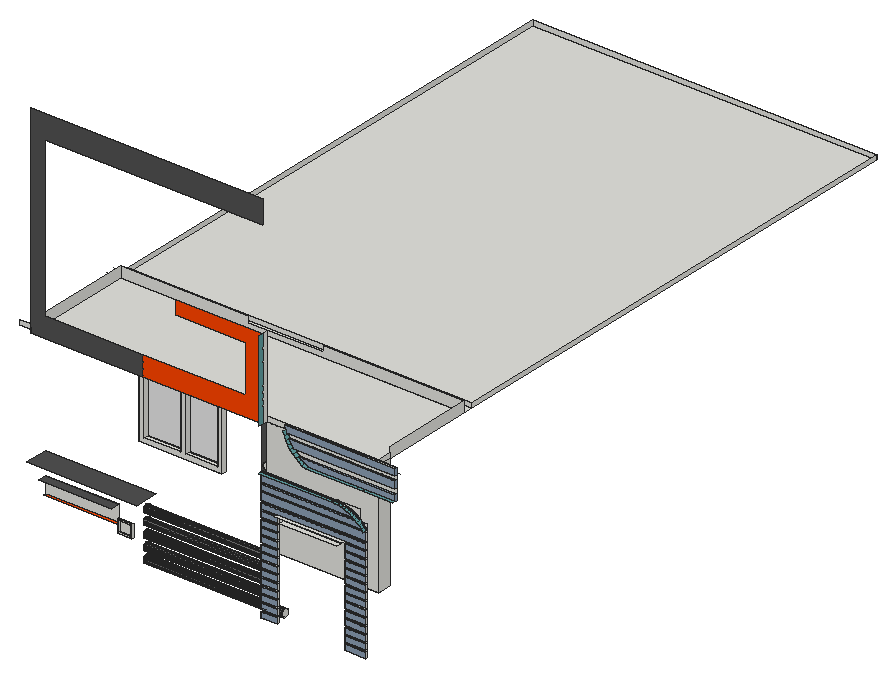
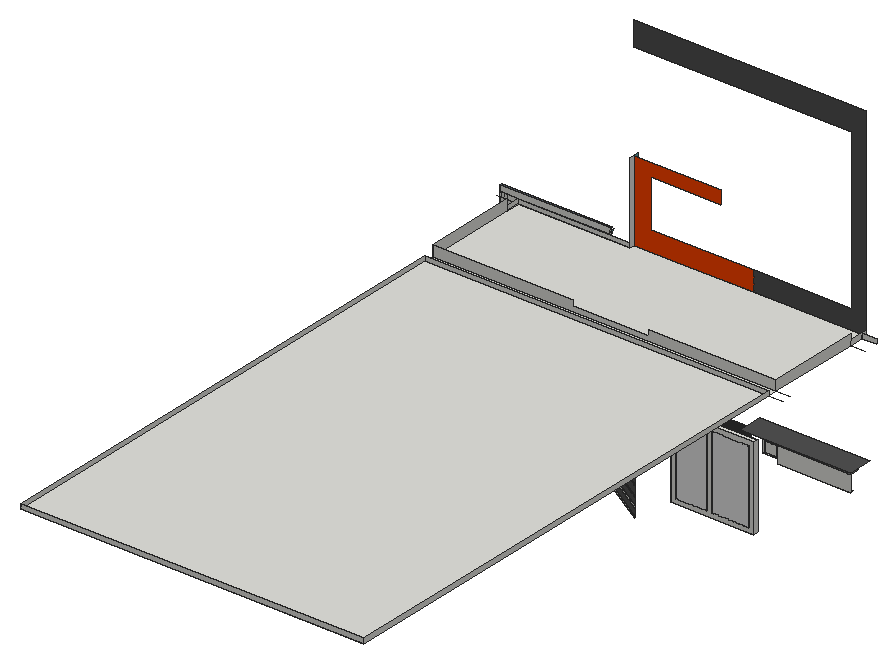
# SketchUp Ruby script. Lengths in inches.
U = 1.inch
M = Sketchup.active_model
def pt(a) = Geom::Point3d.new(a.map { |v| v * U })
def face(e, loops, mat)
  f = e.add_face(loops[0].map { |a| pt(a) })
  loops[1..].each { |l| e.add_face(l.map { |a| pt(a) }).erase! }
  f.material = f.back_material = mat if mat
  f
end
# faces: each face lists its corners as indices into pts; further lists are holes
def faces(e, pts, list, mat = nil) = list.each { |f| face(e, (f[0].is_a?(Array) ? f : [f]).map { |l| l.map { |i| pts[i] } }, mat) }
# xy, xz, yz: faces in a plane at the given z, y or x. An outline is a flat list of corners, or four numbers for a rectangle; further outlines are holes
def ring(l) = l.size == 4 ? [[l[0], l[1]], [l[2], l[1]], [l[2], l[3]], [l[0], l[3]]] : l.each_slice(2).to_a
def flat(e, list, mat, &to3) = list.each { |f| face(e, (f[0].is_a?(Array) ? f : [f]).map { |l| ring(l).map { |u, v| to3.(u, v) } }, mat) }
def xy(e, z, list, mat = nil) = flat(e, list, mat) { |x, y| [x, y, z] }
def xz(e, y, list, mat = nil) = flat(e, list, mat) { |x, z| [x, y, z] }
def yz(e, x, list, mat = nil) = flat(e, list, mat) { |y, z| [x, y, z] }
def lines(e, pts, list) = list.each { |a, b| e.add_line(pt(pts[a]), pt(pts[b])) }
# prism: a flat outline (further loops are holes) pulled along v
def prism(e, loops, v, mat = nil)
  f = face(e, loops, mat); d = Geom::Vector3d.new(v.map { |x| x * U })
  f.pushpull(f.normal.samedirection?(d) ? d.length : -d.length)
end
def box(e, o, s, mat = nil) = prism(e, [[o, [o[0] + s[0], o[1], o[2]], [o[0] + s[0], o[1] + s[1], o[2]], [o[0], o[1] + s[1], o[2]]]], [0, 0, s[2]], mat)
def at(x, y, z, deg = 0) = Geom::Transformation.translation(pt([x, y, z])) * Geom::Transformation.rotation(ORIGIN, Z_AXIS, deg.degrees)
def axes(o, x, y, z) = Geom::Transformation.new([*x, 0, *y, 0, *z, 0, *pt(o).to_a, 1])
def part(name) = M.definitions.add(name)
# library, detail: a bought-in or finely detailed component or shape, given as its bounding box
def library(name, o, s) = part(name).tap { |d| box(d.entities, o, s) }
def detail(e, o, s) = box(e.add_group.entities, o, s)
def put(e, d, t, mat = nil) = e.add_instance(d, t).tap { |i| i.material = mat if mat }
def group(e, t, mat = nil) = e.add_group.tap { |g| g.transformation = t; g.material = mat if mat }.entities
root = M.entities
M.materials.add("[0024_OrangeRed]").color = [255, 69, 0]
M.materials.add("[0081_CadetBlue]").color = [95, 158, 160]
M.materials.add("[0110_LightSlateGray]").color = [139, 158, 178]
M.materials.add("[0134_DimGray]").color = [105, 105, 105]
M.materials.add("[0135_DarkGray]").color = [81, 81, 81]
M.materials.add("[Mirror 02]").color = [229, 229, 229]
xy(root,130.6875,[[213.13,8,226.59,9]])
xy(root,130.6875,[[160.53,8,170.69,9]],"[0110_LightSlateGray]")
xy(root,134.07,[[160.53,8,170.69,9],[213.13,8,226.59,9]],"[0110_LightSlateGray]")
xy(root,135.43,[[213.13,8,226.59,9]])
xy(root,135.43,[[160.53,8,170.69,9]],"[0110_LightSlateGray]")
xy(root,138.8125,[[160.53,8,170.69,9],[213.13,8,226.59,9]],"[0110_LightSlateGray]")
xy(root,140.17,[[213.13,8,226.59,9]])
xy(root,140.17,[[160.53,8,170.69,9]],"[0110_LightSlateGray]")
xy(root,143.55,[[160.53,8,170.69,9],[213.13,8,226.59,9]],"[0110_LightSlateGray]")
xy(root,144.92,[[213.13,8,226.59,9]])
xy(root,144.92,[[160.53,8,170.69,9]],"[0110_LightSlateGray]")
xy(root,148.3,[[160.53,8,170.69,9],[213.13,8,226.59,9]],"[0110_LightSlateGray]")
xy(root,148.91,[[72,5,81.25,6]])
xy(root,149.66,[[213.13,8,226.59,9]])
xy(root,149.66,[[160.53,8,170.69,9]],"[0110_LightSlateGray]")
xy(root,149.71,[[72.8,5,80.45,6]])
xy(root,150.3,[[21.23,10.125,67.5,12]],"[0024_OrangeRed]")
xy(root,153.04,[[160.53,8,170.69,9],[213.13,8,226.59,9]],"[0110_LightSlateGray]")
xy(root,153.81,[[28.3,76.875,80.67,79.875]])
xy(root,154.4,[[213.13,8,226.59,9]])
xy(root,154.4,[[160.53,8,170.69,9]],"[0110_LightSlateGray]")
xy(root,156.24,[[72.8,5,80.45,6]])
xy(root,156.81,[[31.3,76.875,54.48,79.875],[57.67,76.875,77.67,79.875]])
xy(root,157.04,[[72,5,81.25,6]])
xy(root,157.78,[[160.53,8,170.69,9],[213.13,8,226.59,9]],"[0110_LightSlateGray]")
xy(root,159.14,[[213.13,8,226.59,9]])
xy(root,159.14,[[160.53,8,170.69,9]],"[0110_LightSlateGray]")
xy(root,160.4375,[[21.23,6,67.5,12]],"[0135_DarkGray]")
xy(root,162.52,[[160.53,8,170.69,9],[213.13,8,226.59,9]],"[0110_LightSlateGray]")
xy(root,163.88,[[213.13,8,226.59,9]])
xy(root,163.88,[[160.53,8,170.69,9]],"[0110_LightSlateGray]")
xy(root,167.26,[[160.53,8,170.69,9],[213.13,8,226.59,9]],"[0110_LightSlateGray]")
xy(root,168,[[160.53,12,231.375,21]])
xy(root,168,[[14,6,83.4375,21]],"[0135_DarkGray]")
xy(root,168.625,[[213.13,8,226.59,9]])
xy(root,168.625,[[160.53,8,170.69,9]],"[0110_LightSlateGray]")
xy(root,172.01,[[160.53,8,170.69,9],[213.13,8,226.59,9]],"[0110_LightSlateGray]")
xy(root,173.37,[[213.13,8,226.59,9]])
xy(root,173.37,[[160.53,8,170.69,9]],"[0110_LightSlateGray]")
xy(root,176.75,[[160.53,8,170.69,9],[213.13,8,226.59,9]],"[0110_LightSlateGray]")
xy(root,178.11,[[213.13,8,226.59,9]])
xy(root,178.11,[[160.53,8,170.69,9]],"[0110_LightSlateGray]")
xy(root,181.49,[[160.53,8,170.69,9],[213.13,8,226.59,9]],"[0110_LightSlateGray]")
xy(root,182.85,[[213.13,8,226.59,9]])
xy(root,182.85,[[160.53,8,170.69,9]],"[0110_LightSlateGray]")
xy(root,186.23,[[160.53,8,170.69,9],[213.13,8,226.59,9]],"[0110_LightSlateGray]")
xy(root,187.59,[[213.13,8,226.59,9]])
xy(root,187.59,[[160.53,8,170.69,9]],"[0110_LightSlateGray]")
xy(root,189.37,[[173.69,6,210.13,9]])
xy(root,190.98,[[160.53,8,170.69,9],[213.13,8,226.59,9]],"[0110_LightSlateGray]")
xy(root,192.34,[[170.69,6,213.13,9],[213.13,8,226.59,9]])
xy(root,192.34,[[160.53,8,170.69,9]],"[0110_LightSlateGray]")
xy(root,192.37,[[170.69,8,213.13,9]])
xy(root,195.72,[[160.53,8,226.59,9]],"[0110_LightSlateGray]")
xy(root,197.1,[[160.53,8,226.59,9]],"[0110_LightSlateGray]")
xy(root,201,[[105.55,73.875,147.55,76.875]],"[0135_DarkGray]")
xy(root,201.62,[[160.53,8,226.59,9]],"[0110_LightSlateGray]")
xy(root,202.88,[[160.53,8,226.59,9]],"[0110_LightSlateGray]")
xy(root,203.18,[[31.3,76.875,54.48,79.875],[57.67,76.875,77.67,79.875]])
xy(root,204,[[102.55,73.875,150.55,79.875]],"[0135_DarkGray]")
xy(root,206.18,[[28.3,76.875,80.67,79.875]])
xy(root,206.57,[[160.53,8,223.35,9]],"[0110_LightSlateGray]")
xy(root,207.78,[[160.53,8,221.97,9]],"[0110_LightSlateGray]")
xy(root,213.14,[[160.53,8,206.79,9]])
xy(root,213.14,[[160.53,6,206.79,8]],"[0081_CadetBlue]")
xy(root,226.28,[[190.26,8,226.59,9],[226.59,8,245.1875,9]])
xy(root,226.28,[[190.26,6,226.59,8],[226.59,6,240.375,8],[240.375,6,245.1875,8]],"[0081_CadetBlue]")
xy(root,230.16,[[183.95,8,245.1875,9]],"[0110_LightSlateGray]")
xy(root,233.27,[[180.84,8,245.1875,9]],"[0110_LightSlateGray]")
xy(root,237.82,[[177.75,8,245.1875,9]],"[0110_LightSlateGray]")
xy(root,240,[[14,9,14,79.875,231.375,79.875,231.375,12,160.53,12,160.53,9],[14,79.875,231.375,85.875],[14,85.875,231.375,405.4375]])
xy(root,240.67,[[176.48,8,245.1875,9]],"[0110_LightSlateGray]")
xz(root,5,[[[72,148.91,81.25,157.04],[72.8,149.71,80.45,156.24]]])
xz(root,6,[[72.8,149.71,80.45,156.24]])
xz(root,8,[[160.53,130.6875,170.69,134.07],[213.13,130.6875,226.59,134.07],[160.53,135.43,170.69,138.8125],[213.13,135.43,226.59,138.8125],[160.53,140.17,170.69,143.55],
  [213.13,140.17,226.59,143.55],[160.53,144.92,170.69,148.3],[213.13,144.92,226.59,148.3],[160.53,149.66,170.69,153.04],[213.13,149.66,226.59,153.04],
  [160.53,154.4,170.69,157.78],[213.13,154.4,226.59,157.78],[160.53,159.14,170.69,162.52],[213.13,159.14,226.59,162.52],[160.53,163.88,170.69,167.26],
  [213.13,163.88,226.59,167.26],[160.53,168.625,170.69,172.01],[213.13,168.625,226.59,172.01],[160.53,173.37,170.69,176.75],[213.13,173.37,226.59,176.75],
  [160.53,178.11,170.69,181.49],[213.13,178.11,226.59,181.49],[160.53,182.85,170.69,186.23],[213.13,182.85,226.59,186.23],[160.53,187.59,170.69,190.98],
  [213.13,187.59,226.59,190.98],[160.53,192.34,170.69,192.34,170.69,192.37,213.13,192.37,213.13,192.34,226.59,192.34,226.59,195.72,160.53,195.72],[160.53,197.1,226.59,201.62],[160.53,202.88,226.59,202.88,225.42,204.41,224.12,205.84,223.35,206.57,160.53,206.57],[160.53,207.78,221.97,207.78,221.22,208.38,219.62,209.47,217.94,210.42,216.19,211.24,214.39,211.92,212.53,212.45,210.64,212.84,208.72,213.07,206.79,213.14,160.53,213.14],
  [190.26,226.28,245.1875,226.28,245.1875,230.16,183.95,230.16,185.92,228.66,188.03,227.37],[180.84,233.27,245.1875,233.27,245.1875,237.82,177.75,237.82,179.01,235.68,180.47,233.68],[176.48,240.67,245.1875,240.67,245.1875,244.8,175.28,244.8,175.87,242.4]],"[0110_LightSlateGray]")
xz(root,9,[[160.53,130.6875,170.69,134.07],[213.13,130.6875,226.59,134.07],[160.53,134.07,170.69,135.43],[213.13,134.07,226.59,135.43],[160.53,135.43,170.69,138.8125],
  [213.13,135.43,226.59,138.8125],[160.53,138.8125,170.69,140.17],[213.13,138.8125,226.59,140.17],[160.53,140.17,170.69,143.55],[213.13,140.17,226.59,143.55],
  [160.53,143.55,170.69,144.92],[213.13,143.55,226.59,144.92],[160.53,144.92,170.69,148.3],[213.13,144.92,226.59,148.3],[160.53,148.3,170.69,149.66],
  [213.13,148.3,226.59,149.66],[160.53,149.66,170.69,153.04],[213.13,149.66,226.59,153.04],[160.53,153.04,170.69,154.4],[213.13,153.04,226.59,154.4],
  [160.53,154.4,170.69,157.78],[213.13,154.4,226.59,157.78],[160.53,157.78,170.69,159.14],[213.13,157.78,226.59,159.14],[160.53,159.14,170.69,162.52],
  [213.13,159.14,226.59,162.52],[160.53,162.52,170.69,163.88],[213.13,162.52,226.59,163.88],[160.53,163.88,170.69,167.26],[213.13,163.88,226.59,167.26],
  [160.53,167.26,170.69,168.625],[213.13,167.26,226.59,168.625],[160.53,168.625,170.69,172.01],[213.13,168.625,226.59,172.01],[160.53,172.01,170.69,173.37],
  [213.13,172.01,226.59,173.37],[160.53,173.37,170.69,176.75],[213.13,173.37,226.59,176.75],[160.53,176.75,170.69,178.11],[213.13,176.75,226.59,178.11],
  [160.53,178.11,170.69,181.49],[213.13,178.11,226.59,181.49],[160.53,181.49,170.69,182.85],[213.13,181.49,226.59,182.85],[160.53,182.85,170.69,186.23],
  [213.13,182.85,226.59,186.23],[160.53,186.23,170.69,187.59],[213.13,186.23,226.59,187.59],[160.53,187.59,170.69,190.98],[213.13,187.59,226.59,190.98],
  [160.53,190.98,170.69,192.34],[213.13,190.98,226.59,192.34],[160.53,192.34,160.53,195.72,226.59,195.72,226.59,192.34,213.13,192.34,213.13,192.37,170.69,192.37,170.69,192.34],[170.69,192.34,213.13,192.37],[160.53,195.72,226.59,197.1],
  [160.53,197.1,226.59,201.62],[160.53,201.62,226.59,202.88],[160.53,202.88,160.53,206.57,223.35,206.57,224.12,205.84,225.42,204.41,226.59,202.88],[226.59,202.88,226.59,206.57,223.35,206.57,224.12,205.84,225.42,204.41],[160.53,206.57,223.35,206.57,222.72,207.17,221.97,207.78,160.53,207.78],
  [160.53,207.78,160.53,213.14,206.79,213.14,208.72,213.07,210.64,212.84,212.53,212.45,214.39,211.92,216.19,211.24,217.94,210.42,219.62,209.47,221.22,208.38,221.97,207.78],[221.97,207.78,221.97,213.14,206.79,213.14,208.72,213.07,210.64,212.84,212.53,212.45,214.39,211.92,216.19,211.24,217.94,210.42,219.62,209.47,221.22,208.38],[183.95,226.28,190.26,226.28,188.03,227.37,185.92,228.66,183.95,230.16],[190.26,226.28,188.03,227.37,185.92,228.66,183.95,230.16,245.1875,230.16,245.1875,226.28],[183.95,230.16,245.1875,230.16,245.1875,233.27,180.84,233.27,182.125,231.84],
  [177.75,233.27,180.84,233.27,180.47,233.68,179.01,235.68,177.75,237.82],[180.84,233.27,180.47,233.68,179.01,235.68,177.75,237.82,245.1875,237.82,245.1875,233.27],[177.75,237.82,245.1875,237.82,245.1875,240.67,176.48,240.67,176.7,240.0625],[175.28,240.67,176.48,240.67,175.87,242.4,175.28,244.8],[176.48,240.67,175.87,242.4,175.28,244.8,245.1875,244.8,245.1875,240.67]])
xz(root,9,[[85.04,240,160.53,240,160.53,291,105.73,291,105.73,282.37,150.17,282.37,150.17,252.44,85.04,252.44]],"[0024_OrangeRed]")
xz(root,9,[[14,240,85.04,240,85.04,252.44,22.75,252.44,22.75,352.5,160.53,352.5,160.53,367.625,14,367.625]],"[0135_DarkGray]")
xz(root,12,[[21.23,150.3,67.5,160.4375],[160.53,168,231.375,240],[5,240,14,243],[160.53,240,231.375,243],[231.375,240,238.75,243],
  [238.75,240,240.375,243],[240.375,240,241.9375,243]])
xz(root,73.875,[[111.2,167.51,111.84,167.53,112.45,167.71,112.99,168.05,113.42,168.52,113.72,169.08,113.86,169.7,113.84,170.34,113.65,170.94,113.3125,171.48,112.85,171.92,112.29,172.22,111.67,172.36,111.03,172.34,110.42,172.15,109.88,171.8125,109.45,171.35,109.15,170.78,109.01,170.16,109.03,169.53,109.22,168.92,109.55,168.38,110.02,167.95,110.58,167.65]])
xz(root,76.875,[[105.55,134.71,147.55,171.23,147.55,172.96,105.55,135.64],[105.55,140.71,147.55,177.23,147.55,178.96,105.55,141.64],[105.55,146.71,147.55,183.23,147.55,184.96,105.55,147.64],[105.55,152.71,147.55,189.23,147.55,190.96,105.55,153.64],[[28.3,153.81,80.67,206.18],[31.3,156.81,54.48,203.18],[57.67,156.81,77.67,203.18]]])
xz(root,76.875,[[105.55,135.64,147.55,172.96,147.55,177.23,105.55,140.71],[105.55,141.64,147.55,178.96,147.55,183.23,105.55,146.71],[105.55,147.64,147.55,184.96,147.55,189.23,105.55,152.71],[[105.55,153.64,147.55,190.96,147.55,201,105.55,201],[111.2,167.51,110.58,167.65,110.02,167.95,109.55,168.38,109.22,168.92,109.03,169.53,109.01,170.16,109.15,170.78,109.45,171.35,109.88,171.8125,110.42,172.15,111.03,172.34,111.67,172.36,112.29,172.22,112.85,171.92,113.3125,171.48,113.65,170.94,113.84,170.34,113.86,169.7,113.72,169.08,113.42,168.52,112.99,168.05,112.45,167.71,111.84,167.53]]],"[0135_DarkGray]")
xz(root,79.875,[[[28.3,153.81,80.67,206.18],[31.3,156.81,54.48,203.18],[57.67,156.81,77.67,203.18]],[14,240,231.375,240,231.375,246.6875,142.49,246.6875,142.49,243,94.49,243,94.49,246.6875,14,246.6875]])
xz(root,79.875,[[31.3,156.81,54.48,203.18],[57.67,156.81,77.67,203.18]],"[Mirror 02]")
xz(root,85.875,[[14,240,231.375,243]])
xz(root,405.4375,[[14,240,231.375,243]])
yz(root,14,[[9,240,12,243],[12,240,21,243],[21,240,79.875,246.6875],[85.875,240,405.4375,243]])
yz(root,28.3,[[76.875,153.81,79.875,206.18]])
yz(root,31.3,[[76.875,156.81,79.875,203.18]])
yz(root,54.48,[[76.875,156.81,79.875,203.18]])
yz(root,57.67,[[76.875,156.81,79.875,203.18]])
yz(root,72,[[5,148.91,6,157.04]])
yz(root,72.8,[[5,149.71,6,156.24]])
yz(root,77.67,[[76.875,156.81,79.875,203.18]])
yz(root,80.45,[[5,149.71,6,156.24]])
yz(root,80.67,[[76.875,153.81,79.875,206.18]])
yz(root,81.25,[[5,148.91,6,157.04]])
yz(root,160.53,[[9,240,12,291]])
yz(root,160.53,[[6,240,9,291]],"[0081_CadetBlue]")
yz(root,160.53,[[8,130.6875,9,134.07],[8,135.43,9,138.8125],[8,140.17,9,143.55],[8,144.92,9,148.3],[8,149.66,9,153.04],
  [8,154.4,9,157.78],[8,159.14,9,162.52],[8,163.88,9,167.26],[8,168.625,9,172.01],[8,173.37,9,176.75],
  [8,178.11,9,181.49],[8,182.85,9,186.23],[8,187.59,9,190.98],[8,192.34,9,195.72],[8,197.1,9,201.62],
  [8,202.88,9,206.57],[8,207.78,9,213.14]],"[0110_LightSlateGray]")
yz(root,163.375,[[13.48,160.8125,14.06,160.89,14.6,161.11,15.07,161.47,15.42,161.9375,15.65,162.48,15.73,163.0625,15.65,163.64,15.42,164.1875,15.07,164.65,14.6,165.01,14.06,165.23,13.48,165.3125,12.89,165.23,12.35,165.01,11.88,164.65,11.53,164.1875,11.3,163.64,11.23,163.0625,11.3,162.48,11.53,161.9375,11.88,161.47,12.35,161.11,12.89,160.89]])
yz(root,164.1875,[[13.48,153.6875,14.06,153.76,14.6,153.99,15.07,154.34,15.42,154.8125,15.65,155.35,15.73,155.9375,15.65,156.52,15.42,157.0625,15.07,157.53,14.6,157.88,14.06,158.11,13.48,158.1875,12.89,158.11,12.35,157.88,11.88,157.53,11.53,157.0625,11.3,156.52,11.23,155.9375,11.3,155.35,11.53,154.8125,11.88,154.34,12.35,153.99,12.89,153.76]])
yz(root,164.4375,[[13.48,146.5625,14.06,146.64,14.6,146.86,15.07,147.22,15.42,147.6875,15.65,148.23,15.73,148.8125,15.65,149.39,15.42,149.9375,15.07,150.4,14.6,150.76,14.06,150.98,13.48,151.0625,12.89,150.98,12.35,150.76,11.88,150.4,11.53,149.9375,11.3,149.39,11.23,148.8125,11.3,148.23,11.53,147.6875,11.88,147.22,12.35,146.86,12.89,146.64]])
yz(root,164.6875,[[13.48,139.4375,14.06,139.51,14.6,139.74,15.07,140.09,15.42,140.5625,15.65,141.1,15.73,141.6875,15.65,142.27,15.42,142.8125,15.07,143.28,14.6,143.63,14.06,143.86,13.48,143.9375,12.89,143.86,12.35,143.63,11.88,143.28,11.53,142.8125,11.3,142.27,11.23,141.6875,11.3,141.1,11.53,140.5625,11.88,140.09,12.35,139.74,12.89,139.51]])
yz(root,170.69,[[8,130.6875,9,134.07],[8,135.43,9,138.8125],[8,140.17,9,143.55],[8,144.92,9,148.3],[8,149.66,9,153.04],
  [8,154.4,9,157.78],[8,159.14,9,162.52],[8,163.88,9,167.26],[8,168.625,9,172.01],[8,173.37,9,176.75],
  [8,178.11,9,181.49],[8,182.85,9,186.23],[8,187.59,9,190.98],[8,192.34,9,192.37]])
yz(root,171.375,[[13.48,132.3125,14.06,132.39,14.6,132.61,15.07,132.97,15.42,133.4375,15.65,133.98,15.73,134.5625,15.65,135.14,15.42,135.6875,15.07,136.15,14.6,136.51,14.06,136.73,13.48,136.8125,12.89,136.73,12.35,136.51,11.88,136.15,11.53,135.6875,11.3,135.14,11.23,134.5625,11.3,133.98,11.53,133.4375,11.88,132.97,12.35,132.61,12.89,132.39]])
yz(root,213.13,[[8,130.6875,9,134.07],[8,135.43,9,138.8125],[8,140.17,9,143.55],[8,144.92,9,148.3],[8,149.66,9,153.04],
  [8,154.4,9,157.78],[8,159.14,9,162.52],[8,163.88,9,167.26],[8,168.625,9,172.01],[8,173.37,9,176.75],
  [8,178.11,9,181.49],[8,182.85,9,186.23],[8,187.59,9,190.98],[8,192.34,9,192.37]])
yz(root,226.59,[[8,130.6875,9,134.07],[8,135.43,9,138.8125],[8,140.17,9,143.55],[8,144.92,9,148.3],[8,149.66,9,153.04],
  [8,154.4,9,157.78],[8,159.14,9,162.52],[8,163.88,9,167.26],[8,168.625,9,172.01],[8,173.37,9,176.75],
  [8,178.11,9,181.49],[8,182.85,9,186.23],[8,187.59,9,190.98],[8,192.34,9,195.72],[8,197.1,9,201.62]])
yz(root,231.375,[[12,168,21,240],[12,240,21,243],[21,240,79.875,246.6875],[85.875,240,405.4375,243]])
yz(root,245.1875,[[8,226.28,9,230.16],[8,233.27,9,237.82],[8,240.67,9,244.8]],"[0110_LightSlateGray]")
p = [[83.4375,12.89,132.39],[83.4375,13.48,132.3125],[171.375,13.48,132.3125],[171.375,12.89,132.39],[83.4375,14.06,132.39],[171.375,14.06,132.39],
  [83.4375,12.35,132.61],[171.375,12.35,132.61],[83.4375,14.6,132.61],[171.375,14.6,132.61],[83.4375,11.88,132.97],[171.375,11.88,132.97],
  [83.4375,15.07,132.97],[171.375,15.07,132.97],[83.4375,11.53,133.4375],[171.375,11.53,133.4375],[83.4375,15.42,133.4375],[171.375,15.42,133.4375],
  [83.4375,11.3,133.98],[171.375,11.3,133.98],[83.4375,15.65,133.98],[171.375,15.65,133.98],[83.4375,11.23,134.5625],[171.375,11.23,134.5625],
  [83.4375,15.73,134.5625],[171.375,15.73,134.5625],[83.4375,11.3,135.14],[171.375,11.3,135.14],[83.4375,15.65,135.14],[171.375,15.65,135.14],
  [83.4375,11.53,135.6875],[171.375,11.53,135.6875],[83.4375,15.42,135.6875],[171.375,15.42,135.6875],[83.4375,11.88,136.15],[171.375,11.88,136.15],
  [83.4375,15.07,136.15],[171.375,15.07,136.15],[83.4375,12.35,136.51],[171.375,12.35,136.51],[83.4375,14.6,136.51],[171.375,14.6,136.51],
  [83.4375,12.89,136.73],[171.375,12.89,136.73],[83.4375,14.06,136.73],[171.375,14.06,136.73],[83.4375,13.48,136.8125],[171.375,13.48,136.8125],
  [83.4375,12.89,139.51],[83.4375,13.48,139.4375],[164.6875,13.48,139.4375],[164.6875,12.89,139.51],[83.4375,14.06,139.51],[164.6875,14.06,139.51],
  [83.4375,12.35,139.74],[164.6875,12.35,139.74],[83.4375,14.6,139.74],[164.6875,14.6,139.74],[83.4375,11.88,140.09],[164.6875,11.88,140.09],
  [83.4375,15.07,140.09],[164.6875,15.07,140.09],[83.4375,11.53,140.5625],[164.6875,11.53,140.5625],[83.4375,15.42,140.5625],[164.6875,15.42,140.5625],
  [83.4375,11.3,141.1],[164.6875,11.3,141.1],[83.4375,15.65,141.1],[164.6875,15.65,141.1],[83.4375,11.23,141.6875],[164.6875,11.23,141.6875],
  [83.4375,15.73,141.6875],[164.6875,15.73,141.6875],[83.4375,11.3,142.27],[164.6875,11.3,142.27],[83.4375,15.65,142.27],[164.6875,15.65,142.27],
  [83.4375,11.53,142.8125],[164.6875,11.53,142.8125],[83.4375,15.42,142.8125],[164.6875,15.42,142.8125],[83.4375,11.88,143.28],[164.6875,11.88,143.28],
  [83.4375,15.07,143.28],[164.6875,15.07,143.28],[83.4375,12.35,143.63],[164.6875,12.35,143.63],[83.4375,14.6,143.63],[164.6875,14.6,143.63],
  [83.4375,12.89,143.86],[164.6875,12.89,143.86],[83.4375,14.06,143.86],[164.6875,14.06,143.86],[83.4375,13.48,143.9375],[164.6875,13.48,143.9375],
  [83.4375,12.35,146.86],[83.4375,12.89,146.64],[164.4375,12.89,146.64],[164.4375,12.35,146.86],[83.4375,13.48,146.5625],[164.4375,13.48,146.5625],
  [83.4375,14.06,146.64],[164.4375,14.06,146.64],[83.4375,14.6,146.86],[164.4375,14.6,146.86],[83.4375,11.88,147.22],[164.4375,11.88,147.22],
  [83.4375,15.07,147.22],[164.4375,15.07,147.22],[83.4375,11.53,147.6875],[164.4375,11.53,147.6875],[83.4375,15.42,147.6875],[164.4375,15.42,147.6875],
  [83.4375,11.3,148.23],[164.4375,11.3,148.23],[83.4375,15.65,148.23],[164.4375,15.65,148.23],[83.4375,11.23,148.8125],[164.4375,11.23,148.8125],
  [83.4375,15.73,148.8125],[164.4375,15.73,148.8125],[83.4375,11.3,149.39],[164.4375,11.3,149.39],[83.4375,15.65,149.39],[164.4375,15.65,149.39],
  [83.4375,11.53,149.9375],[164.4375,11.53,149.9375],[83.4375,15.42,149.9375],[164.4375,15.42,149.9375],[83.4375,11.88,150.4],[164.4375,11.88,150.4],
  [83.4375,15.07,150.4],[164.4375,15.07,150.4],[83.4375,12.35,150.76],[164.4375,12.35,150.76],[83.4375,14.6,150.76],[164.4375,14.6,150.76],
  [83.4375,12.89,150.98],[164.4375,12.89,150.98],[83.4375,14.06,150.98],[164.4375,14.06,150.98],[83.4375,13.48,151.0625],[164.4375,13.48,151.0625],
  [83.4375,12.89,153.76],[83.4375,13.48,153.6875],[164.1875,13.48,153.6875],[164.1875,12.89,153.76],[83.4375,14.06,153.76],[164.1875,14.06,153.76],
  [83.4375,12.35,153.99],[164.1875,12.35,153.99],[83.4375,14.6,153.99],[164.1875,14.6,153.99],[83.4375,11.88,154.34],[164.1875,11.88,154.34],
  [83.4375,15.07,154.34],[164.1875,15.07,154.34],[83.4375,11.53,154.8125],[164.1875,11.53,154.8125],[83.4375,15.42,154.8125],[164.1875,15.42,154.8125],
  [83.4375,11.3,155.35],[164.1875,11.3,155.35],[83.4375,15.65,155.35],[164.1875,15.65,155.35],[83.4375,11.23,155.9375],[164.1875,11.23,155.9375],
  [83.4375,15.73,155.9375],[164.1875,15.73,155.9375],[83.4375,11.3,156.52],[164.1875,11.3,156.52],[83.4375,15.65,156.52],[164.1875,15.65,156.52],
  [83.4375,11.53,157.0625],[164.1875,11.53,157.0625],[83.4375,15.42,157.0625],[164.1875,15.42,157.0625],[83.4375,11.88,157.53],[164.1875,11.88,157.53],
  [83.4375,15.07,157.53],[164.1875,15.07,157.53],[83.4375,12.35,157.88],[164.1875,12.35,157.88],[83.4375,14.6,157.88],[164.1875,14.6,157.88],
  [83.4375,12.89,158.11],[164.1875,12.89,158.11],[83.4375,14.06,158.11],[164.1875,14.06,158.11],[83.4375,13.48,158.1875],[164.1875,13.48,158.1875],
  [83.4375,12.89,160.89],[83.4375,13.48,160.8125],[163.375,13.48,160.8125],[163.375,12.89,160.89],[83.4375,14.06,160.89],[163.375,14.06,160.89],
  [83.4375,12.35,161.11],[163.375,12.35,161.11],[83.4375,14.6,161.11],[163.375,14.6,161.11],[83.4375,11.88,161.47],[163.375,11.88,161.47],
  [83.4375,15.07,161.47],[163.375,15.07,161.47],[83.4375,11.53,161.9375],[163.375,11.53,161.9375],[83.4375,15.42,161.9375],[163.375,15.42,161.9375],
  [83.4375,11.3,162.48],[163.375,11.3,162.48],[83.4375,15.65,162.48],[163.375,15.65,162.48],[83.4375,11.23,163.0625],[163.375,11.23,163.0625],
  [83.4375,15.73,163.0625],[163.375,15.73,163.0625],[83.4375,11.3,163.64],[163.375,11.3,163.64],[83.4375,15.65,163.64],[163.375,15.65,163.64],
  [83.4375,11.53,164.1875],[163.375,11.53,164.1875],[83.4375,15.42,164.1875],[163.375,15.42,164.1875],[83.4375,11.88,164.65],[163.375,11.88,164.65],
  [83.4375,15.07,164.65],[163.375,15.07,164.65],[83.4375,12.35,165.01],[163.375,12.35,165.01],[83.4375,14.6,165.01],[163.375,14.6,165.01],
  [83.4375,12.89,165.23],[163.375,12.89,165.23],[83.4375,14.06,165.23],[163.375,14.06,165.23],[83.4375,13.48,165.3125],[163.375,13.48,165.3125],
  [110.58,76.875,167.65],[111.2,76.875,167.51],[111.2,73.875,167.51],[110.58,73.875,167.65],[111.84,76.875,167.53],[111.84,73.875,167.53],
  [112.45,76.875,167.71],[112.45,73.875,167.71],[110.02,76.875,167.95],[110.02,73.875,167.95],[112.99,76.875,168.05],[112.99,73.875,168.05],
  [109.55,76.875,168.38],[109.55,73.875,168.38],[113.42,76.875,168.52],[113.42,73.875,168.52],[109.22,76.875,168.92],[109.22,73.875,168.92],
  [113.72,76.875,169.08],[113.72,73.875,169.08],[109.03,76.875,169.53],[109.03,73.875,169.53],[113.86,76.875,169.7],[113.86,73.875,169.7],
  [109.01,76.875,170.16],[109.01,73.875,170.16],[113.84,76.875,170.34],[113.84,73.875,170.34],[109.15,76.875,170.78],[109.15,73.875,170.78],
  [113.65,76.875,170.94],[113.65,73.875,170.94],[109.45,76.875,171.35],[109.45,73.875,171.35],[113.3125,76.875,171.48],[113.3125,73.875,171.48],
  [109.88,76.875,171.8125],[109.88,73.875,171.8125],[112.85,76.875,171.92],[112.85,73.875,171.92],[110.42,76.875,172.15],[110.42,73.875,172.15],
  [112.29,76.875,172.22],[112.29,73.875,172.22],[111.03,76.875,172.34],[111.03,73.875,172.34],[111.67,76.875,172.36],[111.67,73.875,172.36],
  [225.42,6,204.41],[225.42,8,204.41],[226.59,8,202.88],[226.59,6,202.88],[225.42,9,204.41],[226.59,9,202.88],
  [224.12,6,205.84],[224.12,8,205.84],[224.12,9,205.84],[222.72,9,207.17],[223.35,9,206.57],[223.35,8,206.57],
  [222.72,6,207.17],[221.22,6,208.38],[221.22,8,208.38],[221.97,8,207.78],[221.97,9,207.78],[221.22,9,208.38],
  [219.62,6,209.47],[219.62,8,209.47],[219.62,9,209.47],[217.94,6,210.42],[217.94,8,210.42],[217.94,9,210.42],
  [216.19,6,211.24],[216.19,8,211.24],[216.19,9,211.24],[214.39,6,211.92],[214.39,8,211.92],[214.39,9,211.92],
  [212.53,6,212.45],[212.53,8,212.45],[212.53,9,212.45],[210.64,6,212.84],[210.64,8,212.84],[210.64,9,212.84],
  [208.72,6,213.07],[208.72,8,213.07],[208.72,9,213.07],[206.79,6,213.14],[206.79,8,213.14],[206.79,9,213.14],
  [190.26,6,226.28],[190.26,8,226.28],[188.03,8,227.37],[188.03,6,227.37],[190.26,9,226.28],[188.03,9,227.37],
  [185.92,8,228.66],[185.92,6,228.66],[185.92,9,228.66],[183.95,8,230.16],[183.95,6,230.16],[183.95,9,230.16],
  [182.125,9,231.84],[182.125,6,231.84],[180.84,9,233.27],[180.84,8,233.27],[180.47,8,233.68],[180.47,6,233.68],
  [180.47,9,233.68],[179.01,8,235.68],[179.01,6,235.68],[179.01,9,235.68],[177.75,8,237.82],[177.75,6,237.82],
  [177.75,9,237.82],[176.7,9,240.0625],[176.7,6,240.0625],[176.48,9,240.67],[176.48,8,240.67],[175.87,8,242.4],
  [175.87,6,242.4],[175.87,9,242.4],[14,79.875,240],[5,79.875,240],[14,85.875,240],[5,85.875,240],
  [14,21,240],[5,21,240],[231.375,12,240],[231.375,9,240],[241.9375,12,240],[245.1875,12,240]]
faces(root,p,[[0,1,2,3],[1,4,5,2],[6,0,3,7],[4,8,9,5],[10,6,7,11],[8,12,13,9],[14,10,11,15],[12,16,17,13],
  [18,14,15,19],[16,20,21,17],[22,18,19,23],[20,24,25,21],[26,22,23,27],[24,28,29,25],[30,26,27,31],[28,32,33,29],
  [34,30,31,35],[32,36,37,33],[38,34,35,39],[36,40,41,37],[42,38,39,43],[40,44,45,41],[46,42,43,47],[44,46,47,45],
  [48,49,50,51],[49,52,53,50],[54,48,51,55],[52,56,57,53],[58,54,55,59],[56,60,61,57],[62,58,59,63],[60,64,65,61],
  [66,62,63,67],[64,68,69,65],[70,66,67,71],[68,72,73,69],[74,70,71,75],[72,76,77,73],[78,74,75,79],[76,80,81,77],
  [82,78,79,83],[80,84,85,81],[86,82,83,87],[84,88,89,85],[90,86,87,91],[88,92,93,89],[94,90,91,95],[92,94,95,93],
  [96,97,98,99],[97,100,101,98],[100,102,103,101],[102,104,105,103],[106,96,99,107],[104,108,109,105],[110,106,107,111],[108,112,113,109],
  [114,110,111,115],[112,116,117,113],[118,114,115,119],[116,120,121,117],[122,118,119,123],[120,124,125,121],[126,122,123,127],[124,128,129,125],
  [130,126,127,131],[128,132,133,129],[134,130,131,135],[132,136,137,133],[138,134,135,139],[136,140,141,137],[142,138,139,143],[140,142,143,141],
  [144,145,146,147],[145,148,149,146],[150,144,147,151],[148,152,153,149],[154,150,151,155],[152,156,157,153],[158,154,155,159],[156,160,161,157],
  [162,158,159,163],[160,164,165,161],[166,162,163,167],[164,168,169,165],[170,166,167,171],[168,172,173,169],[174,170,171,175],[172,176,177,173],
  [178,174,175,179],[176,180,181,177],[182,178,179,183],[180,184,185,181],[186,182,183,187],[184,188,189,185],[190,186,187,191],[188,190,191,189],
  [192,193,194,195],[193,196,197,194],[198,192,195,199],[196,200,201,197],[202,198,199,203],[200,204,205,201],[206,202,203,207],[204,208,209,205],
  [210,206,207,211],[208,212,213,209],[214,210,211,215],[212,216,217,213],[218,214,215,219],[216,220,221,217],[222,218,219,223],[220,224,225,221],
  [226,222,223,227],[224,228,229,225],[230,226,227,231],[228,232,233,229],[234,230,231,235],[232,236,237,233],[238,234,235,239],[236,238,239,237]],"[0134_DimGray]")
faces(root,p,[[240,241,242,243],[241,244,245,242],[244,246,247,245],[248,240,243,249],[246,250,251,247],[252,248,249,253],[250,254,255,251],[256,252,253,257],
  [254,258,259,255],[260,256,257,261],[258,262,263,259],[264,260,261,265],[262,266,267,263],[268,264,265,269],[266,270,271,267],[272,268,269,273],
  [270,274,275,271],[276,272,273,277],[274,278,279,275],[280,276,277,281],[278,282,283,279],[284,280,281,285],[282,286,287,283],[286,284,285,287],
  [292,293,290,289],[296,292,289,295],[298,296,295,299],[305,304,303,302],[308,305,302,307],[311,308,307,310],[314,311,310,313],[317,314,313,316],
  [320,317,316,319],[323,320,319,322],[326,323,322,325],[329,326,325,328],[334,335,332,331],[335,338,336,332],[338,341,339,336],[344,348,346,345],
  [348,351,349,346],[351,354,352,349],[357,361,359,358]])
faces(root,p,[[288,289,290,291],[294,295,289,288],[297,298,299,295,294,300],[301,302,303,304,297,300],[306,307,302,301],[309,310,307,306],[312,313,310,309],[315,316,313,312],
  [318,319,316,315],[321,322,319,318],[324,325,322,321],[327,328,325,324],[330,331,332,333],[333,332,336,337],[337,336,339,340],[341,342,343,340,339],
  [342,344,345,346,347,343],[347,346,349,350],[350,349,352,353],[354,355,356,353,352],[355,357,358,359,360,356]],"[0081_CadetBlue]")
lines(root,p,[[362,363],[364,365],[366,367],[368,369],[370,371]])
